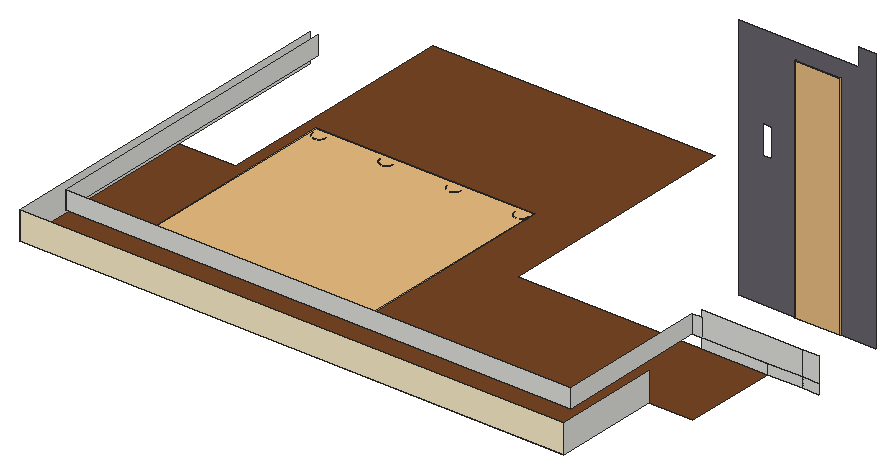
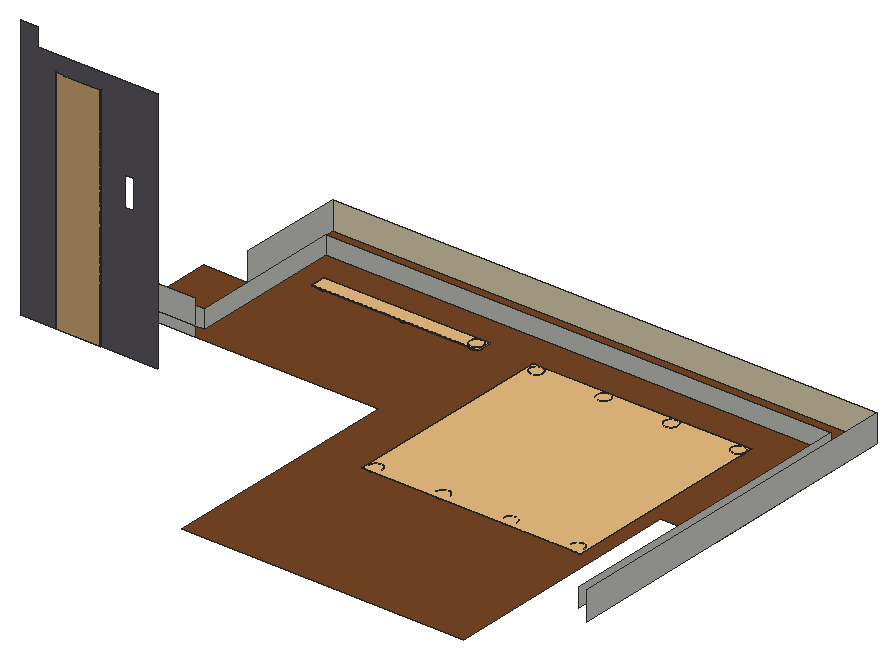
# SketchUp Ruby script. Lengths in inches.
U = 1.inch
M = Sketchup.active_model
def pt(a) = Geom::Point3d.new(a.map { |v| v * U })
def face(e, loops, mat)
  f = e.add_face(loops[0].map { |a| pt(a) })
  loops[1..].each { |l| e.add_face(l.map { |a| pt(a) }).erase! }
  f.material = f.back_material = mat if mat
  f
end
# faces: each face lists its corners as indices into pts; further lists are holes
def faces(e, pts, list, mat = nil) = list.each { |f| face(e, (f[0].is_a?(Array) ? f : [f]).map { |l| l.map { |i| pts[i] } }, mat) }
# xy, xz, yz: faces in a plane at the given z, y or x. An outline is a flat list of corners, or four numbers for a rectangle; further outlines are holes
def ring(l) = l.size == 4 ? [[l[0], l[1]], [l[2], l[1]], [l[2], l[3]], [l[0], l[3]]] : l.each_slice(2).to_a
def flat(e, list, mat, &to3) = list.each { |f| face(e, (f[0].is_a?(Array) ? f : [f]).map { |l| ring(l).map { |u, v| to3.(u, v) } }, mat) }
def xy(e, z, list, mat = nil) = flat(e, list, mat) { |x, y| [x, y, z] }
def xz(e, y, list, mat = nil) = flat(e, list, mat) { |x, z| [x, y, z] }
def yz(e, x, list, mat = nil) = flat(e, list, mat) { |y, z| [x, y, z] }
def lines(e, pts, list) = list.each { |a, b| e.add_line(pt(pts[a]), pt(pts[b])) }
# prism: a flat outline (further loops are holes) pulled along v
def prism(e, loops, v, mat = nil)
  f = face(e, loops, mat); d = Geom::Vector3d.new(v.map { |x| x * U })
  f.pushpull(f.normal.samedirection?(d) ? d.length : -d.length)
end
def box(e, o, s, mat = nil) = prism(e, [[o, [o[0] + s[0], o[1], o[2]], [o[0] + s[0], o[1] + s[1], o[2]], [o[0], o[1] + s[1], o[2]]]], [0, 0, s[2]], mat)
def at(x, y, z, deg = 0) = Geom::Transformation.translation(pt([x, y, z])) * Geom::Transformation.rotation(ORIGIN, Z_AXIS, deg.degrees)
def axes(o, x, y, z) = Geom::Transformation.new([*x, 0, *y, 0, *z, 0, *pt(o).to_a, 1])
def part(name) = M.definitions.add(name)
# library, detail: a bought-in or finely detailed component or shape, given as its bounding box
def library(name, o, s) = part(name).tap { |d| box(d.entities, o, s) }
def detail(e, o, s) = box(e.add_group.entities, o, s)
def put(e, d, t, mat = nil) = e.add_instance(d, t).tap { |i| i.material = mat if mat }
def group(e, t, mat = nil) = e.add_group.tap { |g| g.transformation = t; g.material = mat if mat }.entities
root = M.entities
M.materials.add("[Color D01]").color = [255, 242, 204]
M.materials.add("[Slate Light Tile]").color = [105, 101, 109]
M.materials.add("[Wood Veneer 01]").color = [120, 70, 37]
c1 = library("Group\#19",[-0.5,-0.5,0],[124.4,11,1.0625])
c2 = library("Group\#17",[-0.5,-0.5,-0.1],[163.79,160.18,0.2])
c3 = library("1",[3.97,34.78,0],[101.43,33.99,0.79])
xy(root,252,[[[177.75,359.375,177.75,508.37,220.4375,508.37,220.4375,692.93,431.89,692.93,431.89,508.37,619.25,508.37,619.25,438.56,585.62,438.56,585.62,359.375],[236.74,560.96,238.03,561.13,239.24,561.625,240.27,562.42,241.07,563.46,241.56,564.66,241.74,565.96,241.56,567.25,241.07,568.46,240.27,569.49,239.24,570.29,238.03,570.79,236.74,570.96,235.44,570.79,234.24,570.29,233.2,569.49,232.4,568.46,231.91,567.25,231.74,565.96,231.91,564.66,232.4,563.46,233.2,562.42,234.24,561.625,235.44,561.13],[287.24,560.96,288.53,561.13,289.74,561.625,290.77,562.42,291.57,563.46,292.06,564.66,292.24,565.96,292.06,567.25,291.57,568.46,290.77,569.49,289.74,570.29,288.53,570.79,287.24,570.96,285.94,570.79,284.74,570.29,283.7,569.49,282.9,568.46,282.41,567.25,282.24,565.96,282.41,564.66,282.9,563.46,283.7,562.42,284.74,561.625,285.94,561.13],[337.74,560.96,339.03,561.13,340.24,561.625,341.27,562.42,342.07,563.46,342.56,564.66,342.74,565.96,342.56,567.25,342.07,568.46,341.27,569.49,340.24,570.29,339.03,570.79,337.74,570.96,336.44,570.79,335.24,570.29,334.2,569.49,333.4,568.46,332.91,567.25,332.74,565.96,332.91,564.66,333.4,563.46,334.2,562.42,335.24,561.625,336.44,561.13],[388.24,560.96,389.53,561.13,390.74,561.625,391.77,562.42,392.57,563.46,393.06,564.66,393.24,565.96,393.06,567.25,392.57,568.46,391.77,569.49,390.74,570.29,389.53,570.79,388.24,570.96,386.94,570.79,385.74,570.29,384.7,569.49,383.9,568.46,383.41,567.25,383.24,565.96,383.41,564.66,383.9,563.46,384.7,562.42,385.74,561.625,386.94,561.13],[485.42,409.09,486.71,409.26,487.92,409.76,488.95,410.55,489.75,411.59,490.25,412.8,490.42,414.09,490.25,415.38,489.75,416.59,488.95,417.625,487.92,418.42,486.71,418.92,485.42,419.09,484.125,418.92,482.92,418.42,481.88,417.625,481.09,416.59,480.59,415.38,480.42,414.09,480.59,412.8,481.09,411.59,481.88,410.55,482.92,409.76,484.125,409.26],[434.01,409.09,435.3,409.26,436.51,409.76,437.54,410.55,438.34,411.59,438.84,412.8,439.01,414.09,438.84,415.38,438.34,416.59,437.54,417.625,436.51,418.42,435.3,418.92,434.01,419.09,432.71,418.92,431.51,418.42,430.47,417.625,429.68,416.59,429.18,415.38,429.01,414.09,429.18,412.8,429.68,411.59,430.47,410.55,431.51,409.76,432.71,409.26],[235.44,411.77,236.74,411.94,237.94,412.44,238.98,413.24,239.77,414.27,240.27,415.48,240.44,416.77,240.27,418.07,239.77,419.27,238.98,420.31,237.94,421.1,236.74,421.6,235.44,421.77,234.15,421.6,232.94,421.1,231.91,420.31,231.11,419.27,230.61,418.07,230.44,416.77,230.61,415.48,231.11,414.27,231.91,413.24,232.94,412.44,234.15,411.94],[285.94,411.77,287.24,411.94,288.44,412.44,289.48,413.24,290.27,414.27,290.77,415.48,290.94,416.77,290.77,418.07,290.27,419.27,289.48,420.31,288.44,421.1,287.24,421.6,285.94,421.77,284.65,421.6,283.44,421.1,282.41,420.31,281.61,419.27,281.11,418.07,280.94,416.77,281.11,415.48,281.61,414.27,282.41,413.24,283.44,412.44,284.65,411.94],[336.44,411.77,337.74,411.94,338.94,412.44,339.98,413.24,340.77,414.27,341.27,415.48,341.44,416.77,341.27,418.07,340.77,419.27,339.98,420.31,338.94,421.1,337.74,421.6,336.44,421.77,335.15,421.6,333.94,421.1,332.91,420.31,332.11,419.27,331.61,418.07,331.44,416.77,331.61,415.48,332.11,414.27,332.91,413.24,333.94,412.44,335.15,411.94],[386.94,411.77,388.24,411.94,389.44,412.44,390.48,413.24,391.27,414.27,391.77,415.48,391.94,416.77,391.77,418.07,391.27,419.27,390.48,420.31,389.44,421.1,388.24,421.6,386.94,421.77,385.65,421.6,384.44,421.1,383.41,420.31,382.61,419.27,382.11,418.07,381.94,416.77,382.11,415.48,382.61,414.27,383.41,413.24,384.44,412.44,385.65,411.94],[547.55,409.22,548.8,409.39,549.98,409.875,550.99,410.65,551.76,411.66,552.24,412.83,552.41,414.09,552.24,415.35,551.76,416.52,550.99,417.53,549.98,418.3,548.8,418.79,547.55,418.95,546.29,418.79,545.11,418.3,544.11,417.53,543.33,416.52,542.85,415.35,542.68,414.09,542.85,412.83,543.33,411.66,544.11,410.65,545.11,409.875,546.29,409.39]]],"[Wood Veneer 01]")
xz(root,359.375,[[177.75,252,585.62,273.1875]],"[Color D01]")
xz(root,394.64,[[183.75,259.4375,562.6875,273.1875]])
xz(root,508.37,[[569.82,252,619.25,259.4375],[619.25,252,645.31,259.4375],[645.31,252,657.75,259.4375],[562.6875,259.4375,569.82,273.1875],[569.82,259.4375,645.31,278.125],
  [645.31,259.4375,657.75,278.125]])
xz(root,562.125,[[[554.88,259.4375,597.99,259.4375,597.99,431.7,631.02,431.7,631.02,259.4375,657.75,259.4375,657.75,457.625,644.41,457.625,644.41,444,554.88,444],[572.68,359.15,578.99,381.03]]],"[Slate Light Tile]")
yz(root,177.75,[[359.375,252,631.27,273.1875]])
yz(root,183.75,[[394.64,259.4375,631.27,273.1875]])
yz(root,562.6875,[[394.64,259.4375,508.37,273.1875]])
yz(root,585.62,[[359.375,252,438.56,273.1875]])
p = [[434.01,409.09,252],[432.71,409.26,252],[432.71,409.26,253.9375],[434.01,409.09,253.9375],[435.3,409.26,252],[435.3,409.26,253.9375],
  [485.42,409.09,252],[484.125,409.26,252],[484.125,409.26,252.875],[485.42,409.09,252.875],[486.71,409.26,252],[486.71,409.26,252.875],
  [547.55,409.22,252],[546.29,409.39,252],[546.29,409.39,252.875],[547.55,409.22,252.875],[548.8,409.39,252],[548.8,409.39,252.875],
  [431.51,409.76,252],[431.51,409.76,253.9375],[436.51,409.76,252],[436.51,409.76,253.9375],[482.92,409.76,252],[482.92,409.76,252.875],
  [487.92,409.76,252],[487.92,409.76,252.875],[545.11,409.875,252],[545.11,409.875,252.875],[549.98,409.875,252],[549.98,409.875,252.875],
  [430.47,410.55,252],[430.47,410.55,253.9375],[437.54,410.55,252],[437.54,410.55,253.9375],[481.88,410.55,252],[481.88,410.55,252.875],
  [488.95,410.55,252],[488.95,410.55,252.875],[544.11,410.65,252],[544.11,410.65,252.875],[550.99,410.65,252],[550.99,410.65,252.875],
  [429.68,411.59,252],[429.68,411.59,253.9375],[438.34,411.59,252],[438.34,411.59,253.9375],[481.09,411.59,252],[481.09,411.59,252.875],
  [489.75,411.59,252],[489.75,411.59,252.875],[543.33,411.66,252],[543.33,411.66,252.875],[551.76,411.66,252],[551.76,411.66,252.875],
  [429.18,412.8,252],[429.18,412.8,253.9375],[438.84,412.8,252],[438.84,412.8,253.9375],[480.59,412.8,252],[480.59,412.8,252.875],
  [490.25,412.8,252],[490.25,412.8,252.875],[542.85,412.83,252],[542.85,412.83,252.875],[552.24,412.83,252],[552.24,412.83,252.875],
  [235.44,411.77,252],[234.15,411.94,252],[234.15,411.94,253.1875],[235.44,411.77,253.1875],[236.74,411.94,252],[236.74,411.94,253.1875],
  [285.94,411.77,252],[284.65,411.94,252],[284.65,411.94,253.1875],[285.94,411.77,253.1875],[287.24,411.94,252],[287.24,411.94,253.1875],
  [336.44,411.77,252],[335.15,411.94,252],[335.15,411.94,253.1875],[336.44,411.77,253.1875],[337.74,411.94,252],[337.74,411.94,253.1875],
  [386.94,411.77,252],[385.65,411.94,252],[385.65,411.94,253.1875],[386.94,411.77,253.1875],[388.24,411.94,252],[388.24,411.94,253.1875],
  [232.94,412.44,252],[232.94,412.44,253.1875],[237.94,412.44,252],[237.94,412.44,253.1875],[283.44,412.44,252],[283.44,412.44,253.1875],
  [288.44,412.44,252],[288.44,412.44,253.1875],[333.94,412.44,252],[333.94,412.44,253.1875],[338.94,412.44,252],[338.94,412.44,253.1875],
  [384.44,412.44,252],[384.44,412.44,253.1875],[389.44,412.44,252],[389.44,412.44,253.1875],[231.91,413.24,252],[231.91,413.24,253.1875],
  [238.98,413.24,252],[238.98,413.24,253.1875],[282.41,413.24,252],[282.41,413.24,253.1875],[289.48,413.24,252],[289.48,413.24,253.1875],
  [332.91,413.24,252],[332.91,413.24,253.1875],[339.98,413.24,252],[339.98,413.24,253.1875],[383.41,413.24,252],[383.41,413.24,253.1875],
  [390.48,413.24,252],[390.48,413.24,253.1875],[429.01,414.09,252],[429.01,414.09,253.9375],[439.01,414.09,252],[439.01,414.09,253.9375],
  [480.42,414.09,252],[480.42,414.09,252.875],[490.42,414.09,252],[490.42,414.09,252.875],[542.68,414.09,252],[542.68,414.09,252.875],
  [552.41,414.09,252],[552.41,414.09,252.875],[231.11,414.27,252],[231.11,414.27,253.1875],[239.77,414.27,252],[239.77,414.27,253.1875],
  [281.61,414.27,252],[281.61,414.27,253.1875],[290.27,414.27,252],[290.27,414.27,253.1875],[332.11,414.27,252],[332.11,414.27,253.1875],
  [340.77,414.27,252],[340.77,414.27,253.1875],[382.61,414.27,252],[382.61,414.27,253.1875],[391.27,414.27,252],[391.27,414.27,253.1875],
  [429.18,415.38,252],[429.18,415.38,253.9375],[438.84,415.38,252],[438.84,415.38,253.9375],[480.59,415.38,252],[480.59,415.38,252.875],
  [490.25,415.38,252],[490.25,415.38,252.875],[542.85,415.35,252],[542.85,415.35,252.875],[552.24,415.35,252],[552.24,415.35,252.875],
  [230.61,415.48,252],[230.61,415.48,253.1875],[240.27,415.48,252],[240.27,415.48,253.1875],[281.11,415.48,252],[281.11,415.48,253.1875],
  [290.77,415.48,252],[290.77,415.48,253.1875],[331.61,415.48,252],[331.61,415.48,253.1875],[341.27,415.48,252],[341.27,415.48,253.1875],
  [382.11,415.48,252],[382.11,415.48,253.1875],[391.77,415.48,252],[391.77,415.48,253.1875],[543.33,416.52,252],[543.33,416.52,252.875],
  [551.76,416.52,252],[551.76,416.52,252.875],[429.68,416.59,252],[429.68,416.59,253.9375],[438.34,416.59,252],[438.34,416.59,253.9375],
  [481.09,416.59,252],[481.09,416.59,252.875],[489.75,416.59,252],[489.75,416.59,252.875],[230.44,416.77,252],[230.44,416.77,253.1875],
  [240.44,416.77,252],[240.44,416.77,253.1875],[280.94,416.77,252],[280.94,416.77,253.1875],[290.94,416.77,252],[290.94,416.77,253.1875],
  [331.44,416.77,252],[331.44,416.77,253.1875],[341.44,416.77,252],[341.44,416.77,253.1875],[381.94,416.77,252],[381.94,416.77,253.1875],
  [391.94,416.77,252],[391.94,416.77,253.1875],[544.11,417.53,252],[544.11,417.53,252.875],[550.99,417.53,252],[550.99,417.53,252.875],
  [430.47,417.625,252],[430.47,417.625,253.9375],[437.54,417.625,252],[437.54,417.625,253.9375],[481.88,417.625,252],[481.88,417.625,252.875],
  [488.95,417.625,252],[488.95,417.625,252.875],[230.61,418.07,252],[230.61,418.07,253.1875],[240.27,418.07,252],[240.27,418.07,253.1875],
  [281.11,418.07,252],[281.11,418.07,253.1875],[290.77,418.07,252],[290.77,418.07,253.1875],[331.61,418.07,252],[331.61,418.07,253.1875],
  [341.27,418.07,252],[341.27,418.07,253.1875],[382.11,418.07,252],[382.11,418.07,253.1875],[391.77,418.07,252],[391.77,418.07,253.1875],
  [545.11,418.3,252],[545.11,418.3,252.875],[549.98,418.3,252],[549.98,418.3,252.875],[431.51,418.42,252],[431.51,418.42,253.9375],
  [436.51,418.42,252],[436.51,418.42,253.9375],[482.92,418.42,252],[482.92,418.42,252.875],[487.92,418.42,252],[487.92,418.42,252.875],
  [231.11,419.27,252],[231.11,419.27,253.1875],[239.77,419.27,252],[239.77,419.27,253.1875],[281.61,419.27,252],[281.61,419.27,253.1875],
  [290.27,419.27,252],[290.27,419.27,253.1875],[332.11,419.27,252],[332.11,419.27,253.1875],[340.77,419.27,252],[340.77,419.27,253.1875],
  [382.61,419.27,252],[382.61,419.27,253.1875],[391.27,419.27,252],[391.27,419.27,253.1875],[546.29,418.79,252],[546.29,418.79,252.875],
  [548.8,418.79,252],[548.8,418.79,252.875],[432.71,418.92,252],[432.71,418.92,253.9375],[435.3,418.92,252],[435.3,418.92,253.9375],
  [484.125,418.92,252],[484.125,418.92,252.875],[486.71,418.92,252],[486.71,418.92,252.875],[547.55,418.95,252],[547.55,418.95,252.875],
  [434.01,419.09,252],[434.01,419.09,253.9375],[485.42,419.09,252],[485.42,419.09,252.875],[231.91,420.31,252],[231.91,420.31,253.1875],
  [238.98,420.31,252],[238.98,420.31,253.1875],[282.41,420.31,252],[282.41,420.31,253.1875],[289.48,420.31,252],[289.48,420.31,253.1875],
  [332.91,420.31,252],[332.91,420.31,253.1875],[339.98,420.31,252],[339.98,420.31,253.1875],[383.41,420.31,252],[383.41,420.31,253.1875],
  [390.48,420.31,252],[390.48,420.31,253.1875],[232.94,421.1,252],[232.94,421.1,253.1875],[237.94,421.1,252],[237.94,421.1,253.1875],
  [283.44,421.1,252],[283.44,421.1,253.1875],[288.44,421.1,252],[288.44,421.1,253.1875],[333.94,421.1,252],[333.94,421.1,253.1875],
  [338.94,421.1,252],[338.94,421.1,253.1875],[384.44,421.1,252],[384.44,421.1,253.1875],[389.44,421.1,252],[389.44,421.1,253.1875],
  [234.15,421.6,252],[234.15,421.6,253.1875],[236.74,421.6,252],[236.74,421.6,253.1875],[284.65,421.6,252],[284.65,421.6,253.1875],
  [287.24,421.6,252],[287.24,421.6,253.1875],[335.15,421.6,252],[335.15,421.6,253.1875],[337.74,421.6,252],[337.74,421.6,253.1875],
  [385.65,421.6,252],[385.65,421.6,253.1875],[388.24,421.6,252],[388.24,421.6,253.1875],[235.44,421.77,252],[235.44,421.77,253.1875],
  [285.94,421.77,252],[285.94,421.77,253.1875],[336.44,421.77,252],[336.44,421.77,253.1875],[386.94,421.77,252],[386.94,421.77,253.1875],
  [236.74,560.96,252],[235.44,561.13,252],[235.44,561.13,253.1875],[236.74,560.96,253.1875],[238.03,561.13,252],[238.03,561.13,253.1875],
  [287.24,560.96,252],[285.94,561.13,252],[285.94,561.13,253.1875],[287.24,560.96,253.1875],[288.53,561.13,252],[288.53,561.13,253.1875],
  [337.74,560.96,252],[336.44,561.13,252],[336.44,561.13,253.1875],[337.74,560.96,253.1875],[339.03,561.13,252],[339.03,561.13,253.1875],
  [388.24,560.96,252],[386.94,561.13,252],[386.94,561.13,253.1875],[388.24,560.96,253.1875],[389.53,561.13,252],[389.53,561.13,253.1875],
  [234.24,561.625,252],[234.24,561.625,253.1875],[239.24,561.625,252],[239.24,561.625,253.1875],[284.74,561.625,252],[284.74,561.625,253.1875],
  [289.74,561.625,252],[289.74,561.625,253.1875],[335.24,561.625,252],[335.24,561.625,253.1875],[340.24,561.625,252],[340.24,561.625,253.1875],
  [385.74,561.625,252],[385.74,561.625,253.1875],[390.74,561.625,252],[390.74,561.625,253.1875],[233.2,562.42,252],[233.2,562.42,253.1875],
  [240.27,562.42,252],[240.27,562.42,253.1875],[283.7,562.42,252],[283.7,562.42,253.1875],[290.77,562.42,252],[290.77,562.42,253.1875],
  [334.2,562.42,252],[334.2,562.42,253.1875],[341.27,562.42,252],[341.27,562.42,253.1875],[384.7,562.42,252],[384.7,562.42,253.1875],
  [391.77,562.42,252],[391.77,562.42,253.1875],[232.4,563.46,252],[232.4,563.46,253.1875],[241.07,563.46,252],[241.07,563.46,253.1875],
  [282.9,563.46,252],[282.9,563.46,253.1875],[291.57,563.46,252],[291.57,563.46,253.1875],[333.4,563.46,252],[333.4,563.46,253.1875],
  [342.07,563.46,252],[342.07,563.46,253.1875],[383.9,563.46,252],[383.9,563.46,253.1875],[392.57,563.46,252],[392.57,563.46,253.1875],
  [231.91,564.66,252],[231.91,564.66,253.1875],[241.56,564.66,252],[241.56,564.66,253.1875],[282.41,564.66,252],[282.41,564.66,253.1875],
  [292.06,564.66,252],[292.06,564.66,253.1875],[332.91,564.66,252],[332.91,564.66,253.1875],[342.56,564.66,252],[342.56,564.66,253.1875],
  [383.41,564.66,252],[383.41,564.66,253.1875],[393.06,564.66,252],[393.06,564.66,253.1875],[231.74,565.96,252],[231.74,565.96,253.1875],
  [241.74,565.96,252],[241.74,565.96,253.1875],[282.24,565.96,252],[282.24,565.96,253.1875],[292.24,565.96,252],[292.24,565.96,253.1875],
  [332.74,565.96,252],[332.74,565.96,253.1875],[342.74,565.96,252],[342.74,565.96,253.1875],[383.24,565.96,252],[383.24,565.96,253.1875],
  [393.24,565.96,252],[393.24,565.96,253.1875]]
faces(root,p,[[0,1,2,3],[4,0,3,5],[6,7,8,9],[10,6,9,11],[12,13,14,15],[16,12,15,17],[1,18,19,2],[20,4,5,21],
  [7,22,23,8],[24,10,11,25],[13,26,27,14],[28,16,17,29],[18,30,31,19],[32,20,21,33],[22,34,35,23],[36,24,25,37],
  [26,38,39,27],[40,28,29,41],[30,42,43,31],[44,32,33,45],[34,46,47,35],[48,36,37,49],[38,50,51,39],[52,40,41,53],
  [42,54,55,43],[56,44,45,57],[46,58,59,47],[60,48,49,61],[50,62,63,51],[64,52,53,65],[66,67,68,69],[70,66,69,71],
  [72,73,74,75],[76,72,75,77],[78,79,80,81],[82,78,81,83],[84,85,86,87],[88,84,87,89],[67,90,91,68],[92,70,71,93],
  [73,94,95,74],[96,76,77,97],[79,98,99,80],[100,82,83,101],[85,102,103,86],[104,88,89,105],[90,106,107,91],[108,92,93,109],
  [94,110,111,95],[112,96,97,113],[98,114,115,99],[116,100,101,117],[102,118,119,103],[120,104,105,121],[54,122,123,55],[124,56,57,125],
  [58,126,127,59],[128,60,61,129],[62,130,131,63],[132,64,65,133],[106,134,135,107],[136,108,109,137],[110,138,139,111],[140,112,113,141],
  [114,142,143,115],[144,116,117,145],[118,146,147,119],[148,120,121,149],[122,150,151,123],[152,124,125,153],[126,154,155,127],[156,128,129,157],
  [130,158,159,131],[160,132,133,161],[134,162,163,135],[164,136,137,165],[138,166,167,139],[168,140,141,169],[142,170,171,143],[172,144,145,173],
  [146,174,175,147],[176,148,149,177],[158,178,179,159],[180,160,161,181],[150,182,183,151],[184,152,153,185],[154,186,187,155],[188,156,157,189],
  [162,190,191,163],[192,164,165,193],[166,194,195,167],[196,168,169,197],[170,198,199,171],[200,172,173,201],[174,202,203,175],[204,176,177,205],
  [178,206,207,179],[208,180,181,209],[182,210,211,183],[212,184,185,213],[186,214,215,187],[216,188,189,217],[190,218,219,191],[220,192,193,221],
  [194,222,223,195],[224,196,197,225],[198,226,227,199],[228,200,201,229],[202,230,231,203],[232,204,205,233],[206,234,235,207],[236,208,209,237],
  [210,238,239,211],[240,212,213,241],[214,242,243,215],[244,216,217,245],[218,246,247,219],[248,220,221,249],[222,250,251,223],[252,224,225,253],
  [226,254,255,227],[256,228,229,257],[230,258,259,231],[260,232,233,261],[234,262,263,235],[264,236,237,265],[238,266,267,239],[268,240,241,269],
  [242,270,271,243],[272,244,245,273],[262,274,275,263],[274,264,265,275],[266,276,277,267],[276,268,269,277],[270,278,279,271],[278,272,273,279],
  [246,280,281,247],[282,248,249,283],[250,284,285,251],[286,252,253,287],[254,288,289,255],[290,256,257,291],[258,292,293,259],[294,260,261,295],
  [280,296,297,281],[298,282,283,299],[284,300,301,285],[302,286,287,303],[288,304,305,289],[306,290,291,307],[292,308,309,293],[310,294,295,311],
  [296,312,313,297],[314,298,299,315],[300,316,317,301],[318,302,303,319],[304,320,321,305],[322,306,307,323],[308,324,325,309],[326,310,311,327],
  [312,328,329,313],[328,314,315,329],[316,330,331,317],[330,318,319,331],[320,332,333,321],[332,322,323,333],[324,334,335,325],[334,326,327,335],
  [336,337,338,339],[340,336,339,341],[342,343,344,345],[346,342,345,347],[348,349,350,351],[352,348,351,353],[354,355,356,357],[358,354,357,359],
  [337,360,361,338],[362,340,341,363],[343,364,365,344],[366,346,347,367],[349,368,369,350],[370,352,353,371],[355,372,373,356],[374,358,359,375],
  [360,376,377,361],[378,362,363,379],[364,380,381,365],[382,366,367,383],[368,384,385,369],[386,370,371,387],[372,388,389,373],[390,374,375,391],
  [376,392,393,377],[394,378,379,395],[380,396,397,381],[398,382,383,399],[384,400,401,385],[402,386,387,403],[388,404,405,389],[406,390,391,407],
  [392,408,409,393],[410,394,395,411],[396,412,413,397],[414,398,399,415],[400,416,417,401],[418,402,403,419],[404,420,421,405],[422,406,407,423],
  [408,424,425,409],[426,410,411,427],[412,428,429,413],[430,414,415,431],[416,432,433,417],[434,418,419,435],[420,436,437,421],[438,422,423,439]])
put(root,c1,at(429.01,409.09,252.875))
put(root,c2,at(230.44,411.77,253.1875))
put(root,c3,axes([665.8,562.125,252.68],[0,0,1.7],[-1,0,0],[0,-1,0]))
